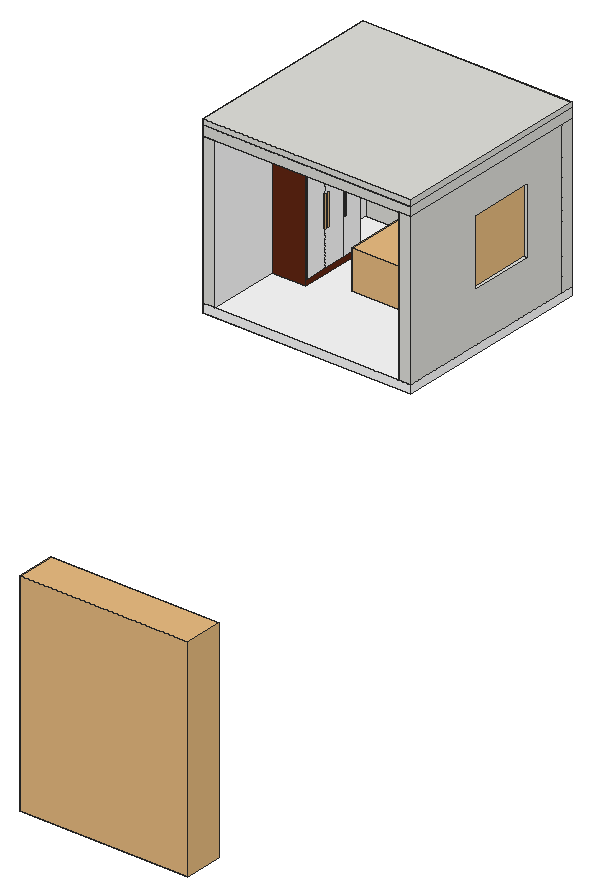
# SketchUp Ruby script. Lengths in inches.
U = 1.inch
M = Sketchup.active_model
def pt(a) = Geom::Point3d.new(a.map { |v| v * U })
def face(e, loops, mat)
  f = e.add_face(loops[0].map { |a| pt(a) })
  loops[1..].each { |l| e.add_face(l.map { |a| pt(a) }).erase! }
  f.material = f.back_material = mat if mat
  f
end
# faces: each face lists its corners as indices into pts; further lists are holes
def faces(e, pts, list, mat = nil) = list.each { |f| face(e, (f[0].is_a?(Array) ? f : [f]).map { |l| l.map { |i| pts[i] } }, mat) }
# xy, xz, yz: faces in a plane at the given z, y or x. An outline is a flat list of corners, or four numbers for a rectangle; further outlines are holes
def ring(l) = l.size == 4 ? [[l[0], l[1]], [l[2], l[1]], [l[2], l[3]], [l[0], l[3]]] : l.each_slice(2).to_a
def flat(e, list, mat, &to3) = list.each { |f| face(e, (f[0].is_a?(Array) ? f : [f]).map { |l| ring(l).map { |u, v| to3.(u, v) } }, mat) }
def xy(e, z, list, mat = nil) = flat(e, list, mat) { |x, y| [x, y, z] }
def xz(e, y, list, mat = nil) = flat(e, list, mat) { |x, z| [x, y, z] }
def yz(e, x, list, mat = nil) = flat(e, list, mat) { |y, z| [x, y, z] }
def lines(e, pts, list) = list.each { |a, b| e.add_line(pt(pts[a]), pt(pts[b])) }
# prism: a flat outline (further loops are holes) pulled along v
def prism(e, loops, v, mat = nil)
  f = face(e, loops, mat); d = Geom::Vector3d.new(v.map { |x| x * U })
  f.pushpull(f.normal.samedirection?(d) ? d.length : -d.length)
end
def box(e, o, s, mat = nil) = prism(e, [[o, [o[0] + s[0], o[1], o[2]], [o[0] + s[0], o[1] + s[1], o[2]], [o[0], o[1] + s[1], o[2]]]], [0, 0, s[2]], mat)
def at(x, y, z, deg = 0) = Geom::Transformation.translation(pt([x, y, z])) * Geom::Transformation.rotation(ORIGIN, Z_AXIS, deg.degrees)
def axes(o, x, y, z) = Geom::Transformation.new([*x, 0, *y, 0, *z, 0, *pt(o).to_a, 1])
def part(name) = M.definitions.add(name)
# library, detail: a bought-in or finely detailed component or shape, given as its bounding box
def library(name, o, s) = part(name).tap { |d| box(d.entities, o, s) }
def detail(e, o, s) = box(e.add_group.entities, o, s)
def put(e, d, t, mat = nil) = e.add_instance(d, t).tap { |i| i.material = mat if mat }
def group(e, t, mat = nil) = e.add_group.tap { |g| g.transformation = t; g.material = mat if mat }.entities
root = M.entities
M.materials.add("Ceramic Sand 8.13cm").color = [255, 255, 255]
M.materials.add("Emissive").color = [255, 202, 141]
M.materials.add("Emissive\#1").color = [255, 201, 138]
M.materials.add("Marble White 501 36.79cm").color = [255, 255, 255]
M.materials.add("Marble White 601 37.77cm\#1").color = [255, 255, 255]
M.materials.add("Wood Dark 02 100cm\#1").color = [99, 39, 19]
M.materials.add("[Color M09]4").color = [0, 0, 0]
M.materials.add("tecido").color = [198, 192, 183]
c1 = part("232mm Slimline Handle")
detail(c1.entities,[0,0,0],[9.13,0.47,1.38])
c2 = library("Double bed set",[6.09,0.88,0],[81.44,100.66,42.94])
c3 = library("Roman blind",[0,0,0],[2.24,37.33,21.19])
c4 = library("Window Crafter Sliding 2",[0,-0.07,0],[48,3.52,48])
c5 = library("Tlon Light 650 Ceiling 152 007",[-12.8,-12.8,-3.78],[25.6,25.6,3.58])
c6 = library("alpha",[-9.58,-11.73,2.09],[20.31,19.05,9.62])
c7 = library("Group\#10",[0,0,9.46],[84,1,110.54])
c8 = library("Group\#9",[0,0,0],[15.0625,1.3125,59.625])
c9 = part("Group\#353")
detail(c9.entities,[0,0,0],[1.58,1.18,1.58])
detail(root,[303.51,0,24.09],[120.56,27.875,151.41])
put(root,c1,axes([34,609.46,59.9],[0,0,-2.46],[0,1,0],[1,0,0]),"[Color M09]4")
put(root,c1,axes([34,627.9375,59.84],[0,0,-2.46],[0,1,0],[1,0,0]),"[Color M09]4")
put(root,c1,axes([34,612.23,59.66],[0,0,-2.46],[0,1,0],[1,0,0]),"[Color M09]4")
put(root,c2,axes([56.36,683.34,6],[0,-0.87706,0],[0.72394,0,0],[0,0,0.65]))
put(root,c3,axes([138.76,600.57,61.6],[1,0,0],[0,1.29,0],[0,0,1.34]),"tecido")
put(root,c4,at(143.81,648.57,42,-90))
put(root,c5,axes([40.37,556.16,114],[0.2,0,0],[0,0.2,0],[0,0,0.2]))
put(root,c5,axes([135.87,556.16,114],[0.2,0,0],[0,0.2,0],[0,0,0.2]))
put(root,c5,axes([135.87,665.54,114],[0.2,0,0],[0,0.2,0],[0,0,0.2]))
put(root,c5,axes([40.37,665.54,114],[0.2,0,0],[0,0.2,0],[0,0,0.2]))
put(root,c6,axes([87.5,610.64,98.94],[1,0,0],[0,1,0],[0,0,1.467]))
g1 = group(root,at(0,543.57,0))
box(g1,[0,0,0],[150,144,6],"Marble White 601 37.77cm\#1")
g2 = group(root,at(0,543.57,6))
xy(g2,0,[[0,0,9,135]])
xy(g2,108,[[0,0,9,135]])
xz(g2,0,[[0,0,9,108]])
xz(g2,135,[[0,0,9,108]])
yz(g2,0,[[0,0,135,108]])
yz(g2,9,[[0,0,135,108]],"Ceramic Sand 8.13cm")
g3 = group(root,at(9,594.57,6))
g4 = group(g3,at(24,0,5.09))
xy(g4,0,[[0,0,1,16.32],[0,16.64,1,32.09],[0,32.41,1,48.02]])
xy(g4,77.08,[[0,83.29,1,84]])
xy(g4,77.5,[[0,16.32,1,16.64],[0,32.09,1,32.41],[0,48.02,1,83.29]])
xy(g4,78.21,[[0,17.07,1,17.38],[0,33.58,1,33.9],[0,50.1,1,50.42],[0.0625,66.62,1,66.93]])
xy(g4,102.91,[[0,0,1,17.07],[0,17.38,1,33.58],[0,33.9,1,50.1],[0,50.42,1,50.42,1,66.62,0.0625,66.62,0.0625,66.93,1,66.93,1,84,0,84]],"Wood Dark 02 100cm\#1")
xz(g4,0,[[0,0,1,102.91]],"Wood Dark 02 100cm\#1")
xz(g4,16.32,[[0,0,1,77.5]])
xz(g4,16.64,[[0,0,1,77.5]])
xz(g4,17.07,[[0,78.21,1,102.21],[0,102.21,1,102.91]])
xz(g4,17.38,[[0,78.21,1,102.21],[0,102.21,1,102.91]])
xz(g4,32.09,[[0,0,1,77.5]])
xz(g4,32.41,[[0,0,1,77.5]])
xz(g4,33.58,[[0,78.21,1,102.21],[0,102.21,1,102.91]])
xz(g4,33.9,[[0,78.21,1,102.21],[0,102.21,1,102.91]])
xz(g4,48.02,[[0,0,1,77.5]])
xz(g4,50.1,[[0,78.21,1,102.21],[0,102.21,1,102.91]])
xz(g4,50.42,[[0,78.21,1,102.21],[0,102.21,1,102.91]])
xz(g4,66.62,[[0.0625,78.21,1,102.21],[0.0625,102.21,1,102.91]])
xz(g4,66.93,[[0.0625,78.21,1,102.21],[0.0625,102.21,1,102.91]])
xz(g4,83.29,[[0,77.08,1,77.5]])
xz(g4,84,[[0,77.08,1,102.91]])
yz(g4,0,[[0,0,0,102.91,17.07,102.91,17.07,78.21,17.38,78.21,17.38,102.91,33.58,102.91,33.58,78.21,33.9,78.21,33.9,102.91,50.1,102.91,50.1,78.21,50.42,78.21,50.42,102.91,84,102.91,84,77.08,83.29,77.08,83.29,77.5,48.02,77.5,48.02,0,32.41,0,32.41,77.5,32.09,77.5,32.09,0,16.64,0,16.64,77.5,16.32,77.5,16.32,0]])
yz(g4,0.0625,[[66.62,78.21,66.93,102.91]])
yz(g4,1,[[83.29,77.08,84,102.21],[83.29,102.21,84,102.91]])
yz(g4,1,[[0.71,0,16.32,77.5],[16.64,0,32.09,77.5],[32.41,0,48.02,77.5],[0.71,78.21,17.07,102.21],[17.38,78.21,33.58,102.21],
  [33.9,78.21,50.1,102.21],[50.42,78.21,66.62,102.21],[66.93,78.21,83.29,102.21]],"Marble White 501 36.79cm")
yz(g4,1,[[0,0,0.71,102.21],[0.71,77.5,83.29,78.21],[0,102.21,0.71,102.91],[0.71,102.21,17.07,102.91],[17.38,102.21,33.58,102.91],
  [33.9,102.21,50.1,102.91],[50.42,102.21,66.62,102.91],[66.93,102.21,83.29,102.91]],"Wood Dark 02 100cm\#1")
p = [[0,84,77.23],[1,83.29,77.08]]
lines(g4,p,[[0,1]])
g5 = group(g3,at(0,0,0))
xy(g5,0,[[0,0,24,48]],"Wood Dark 02 100cm\#1")
xy(g5,82.3125,[[0,48,24,84]],"Wood Dark 02 100cm\#1")
xy(g5,108,[[0,0,24,84]],"Wood Dark 02 100cm\#1")
xz(g5,0,[[0,0,24,108]],"Wood Dark 02 100cm\#1")
xz(g5,48,[[0,0,24,82.3125]],"Wood Dark 02 100cm\#1")
xz(g5,84,[[0,82.3125,24,108]],"Wood Dark 02 100cm\#1")
yz(g5,0,[[0,0,0,108,84,108,84,82.3125,48,82.3125,48,0]],"Wood Dark 02 100cm\#1")
yz(g5,24,[[0,0,47.69,108],[47.69,0,48,108],[48,82.3125,84,108]],"Wood Dark 02 100cm\#1")
put(root,c7,axes([57,676.57,8.4],[1,0,0],[0,1,0],[0,0,0.88]),"Wood Dark 02 100cm\#1")
put(root,c8,axes([37.8125,676.26,29.3],[1,0,0],[0,1,0],[0,0,0.88]))
put(root,c9,axes([35.18,610.64,96.31],[0,-1,0],[-1,0,0],[0,0,-1]))
put(root,c9,axes([35.18,614.33,96.31],[0,-1,0],[-1,0,0],[0,0,-1]))
put(root,c9,axes([35.18,631.05,96.31],[0,-1,0],[-1,0,0],[0,0,-1]))
put(root,c9,axes([35.18,664.09,96.31],[0,-1,0],[-1,0,0],[0,0,-1]))
put(root,c9,axes([35.18,660.16,96.31],[0,-1,0],[-1,0,0],[0,0,-1]))
g6 = group(root,at(0,678.57,6))
box(g6,[0,0,0],[150,9,108])
g7 = group(root,at(141,543.57,6))
xy(g7,0,[[0,0,9,135]])
xy(g7,36,[[0,57,9,105]])
xy(g7,84,[[0,57,9,105]])
xy(g7,108,[[0,0,9,135]])
xz(g7,0,[[0,0,9,108]])
xz(g7,57,[[0,36,9,84]])
xz(g7,105,[[0,36,9,84]])
xz(g7,135,[[0,0,9,108]])
yz(g7,0,[[[0,0,135,108],[57,36,105,84]]],"Ceramic Sand 8.13cm")
yz(g7,9,[[[0,0,135,108],[57,36,105,84]]])
g8 = group(root,at(0,543.57,114))
xy(g8,0,[[0,0,0,144,150,144,150,0,141,0,141,134,34,134,34,0],[[34,0,141,134],[46,12,129,122]]])
xy(g8,2.125,[[58,24,117,110]])
xy(g8,4,[[[40.37,6.37,134.63,127.63],[46,12,129,122]],[[58,24,117,110],[62.67,28.67,112.33,105.33]]],"Emissive\#1")
xy(g8,7,[[[0,0,150,144],[40.37,6.37,134.63,127.63]],[62.67,28.67,112.33,105.33]])
xz(g8,0,[[0,0,150,7]])
xz(g8,6.37,[[40.37,4,134.63,7]])
xz(g8,12,[[46,0,129,4]])
xz(g8,24,[[58,2.125,117,4]])
xz(g8,28.67,[[62.67,4,112.33,7]])
xz(g8,105.33,[[62.67,4,112.33,7]])
xz(g8,110,[[58,2.125,117,4]])
xz(g8,122,[[46,0,129,4]])
xz(g8,127.63,[[40.37,4,134.63,7]])
xz(g8,144,[[0,0,150,7]])
yz(g8,0,[[0,0,144,7]])
yz(g8,40.37,[[6.37,4,127.63,7]])
yz(g8,46,[[12,0,122,4]])
yz(g8,58,[[24,2.125,110,4]])
yz(g8,62.67,[[28.67,4,105.33,7]])
yz(g8,112.33,[[28.67,4,105.33,7]])
yz(g8,117,[[24,2.125,110,4]])
yz(g8,129,[[12,0,122,4]])
yz(g8,134.63,[[6.37,4,127.63,7]])
yz(g8,150,[[0,0,144,7]])
g9 = group(root,at(0,543.57,121))
box(g9,[0,0,0],[150,144,4])
g10 = group(root,at(34,677.57,8.4))
xy(g10,0,[[0,0,107,1]])
xy(g10,105.6,[[0,0,107,1]])
xz(g10,0,[[0,0,107,0,107,1.13,105.69,8.18,105.61,8.76,105.52,9.32,105.43,9.89,105.33,10.45,105.22,11.02,104.98,12.14,104.85,12.7,104.71,13.26,104.5625,13.8125,104.41,14.37,104.09,15.47,103.92,16.03,103.74,16.57,103.36,17.67,103.16,18.21,102.74,19.29,102.52,19.83,102.29,20.36,102.06,20.9,101.82,21.43,101.57,21.96,101.3125,22.48,101.05,23,100.79,23.53,100.51,24.04,100.23,24.56,99.95,25.07,99.35,26.09,99.05,26.59,98.74,27.09,98.42,27.59,98.09,28.09,97.43,29.07,96.38,30.51,96.02,30.98,95.65,31.46,95.28,31.92,94.9,32.39,94.51,32.85,94.12,33.3,93.73,33.76,93.32,34.2,92.92,34.65,92.08,35.53,91.66,35.96,91.23,36.39,90.8,36.8125,90.36,37.23,89.91,37.65,89.46,38.06,89,38.46,88.54,38.87,88.08,39.26,87.61,39.66,87.13,40.05,86.65,40.43,86.16,40.81,85.18,41.55,84.68,41.92,84.17,42.28,83.67,42.63,83.15,42.98,82.64,43.33,82.11,43.67,81.59,44,81.06,44.33,80.52,44.66,79.98,44.98,78.9,45.6,78.35,45.9,77.79,46.2,76.67,46.78,76.11,47.0625,75.54,47.34,74.97,47.61,73.23,48.39,72.65,48.63,72.06,48.875,71.47,49.11,70.28,49.57,69.68,49.79,69.08,50,68.47,50.21,67.86,50.41,66.03,50.98,65.41,51.15,64.79,51.33,63.55,51.65,62.29,51.95,61.03,52.23,60.4,52.36,59.77,52.48,58.49,52.7,57.86,52.81,57.22,52.91,56.58,53,55.93,53.08,55.29,53.16,54.64,53.24,54.2,53.29,53.75,53.34,53.3,53.4,52.85,53.47,52.41,53.54,51.96,53.61,51.52,53.69,51.08,53.78,50.63,53.86,49.75,54.06,49.32,54.16,48.88,54.27,48.45,54.38,48.01,54.5,47.15,54.74,46.72,54.87,46.3,55.01,45.87,55.15,45.45,55.29,44.61,55.59,44.19,55.75,43.78,55.91,42.55,56.42,42.15,56.6,41.74,56.79,41.34,56.97,40.95,57.17,40.55,57.36,40.16,57.5625,39.77,57.77,39.38,57.98,39,58.1875,38.62,58.41,38.24,58.625,37.87,58.85,37.5,59.08,37.13,59.3125,36.77,59.55,36.4,59.79,36.05,60.03,35.69,60.28,35.34,60.53,34.99,60.79,34.65,61.05,34.31,61.3125,33.97,61.58,33.31,62.12,32.98,62.4,32.34,62.96,31.41,63.83,30.81,64.43,30.51,64.74,30.22,65.04,29.9375,65.35,29.66,65.66,29.38,65.98,28.84,66.62,28.58,66.94,28.32,67.27,28.0625,67.6,27.81,67.93,27.5625,68.27,27.32,68.6,27.09,68.94,26.85,69.29,26.63,69.63,26.41,69.98,26.1875,70.33,25.97,70.68,25.77,71.04,25.5625,71.39,25.37,71.75,25.17,72.11,24.98,72.47,24.62,73.21,24.45,73.57,24.28,73.94,24.12,74.32,23.96,74.69,23.81,75.07,23.66,75.44,23.38,76.2,23.25,76.58,23.12,76.97,23,77.35,22.88,77.74,22.77,78.12,22.47,79.29,22.38,79.68,22.22,80.46,22.14,80.86,22.08,81.25,22.01,81.65,21.96,82.04,21.9,82.4375,21.86,82.83,21.78,83.63,21.75,84.03,21.73,84.43,21.71,84.82,21.69,85.22,21.69,85.62,21.68,86.02,21.68,105.6,0,105.6]],"Ceramic Sand 8.13cm")
xz(g10,0,[[107,1.13,107,8.33,106.92,8.91,106.83,9.49,106.73,10.0625,106.625,10.64,106.51,11.22,106.4,11.79,106.27,12.36,106.14,12.9375,105.99,13.51,105.85,14.08,105.69,14.65,105.53,15.21,105.36,15.78,105,16.9,104.8125,17.46,104.61,18.02,104.41,18.57,104.2,19.13,103.98,19.68,103.52,20.78,103.04,21.86,102.26,23.48,101.7,24.54,101.42,25.06,101.125,25.59,100.83,26.11,100.52,26.63,100.21,27.14,99.89,27.66,99.5625,28.17,99.23,28.67,98.55,29.67,98.2,30.17,97.48,31.15,97.11,31.64,96.73,32.12,96.35,32.59,95.96,33.07,95.57,33.54,95.17,34.01,94.35,34.93,93.9375,35.38,93.51,35.83,93.09,36.28,92.21,37.16,91.77,37.59,91.32,38.02,90.86,38.45,90.4,38.87,89.9375,39.28,89.47,39.69,88.99,40.1,88.51,40.5,88.02,40.9,87.53,41.29,87.03,41.68,86.53,42.0625,86.03,42.44,85.51,42.81,85,43.18,84.48,43.55,83.95,43.9,83.43,44.26,82.89,44.6,82.35,44.95,81.8125,45.28,81.27,45.61,80.71,45.94,80.16,46.26,79.6,46.58,79.04,46.89,77.33,47.79,76.75,48.07,76.17,48.36,75.59,48.63,74.41,49.17,73.8125,49.43,73.21,49.68,72.61,49.93,72.01,50.17,71.4,50.41,70.79,50.64,70.18,50.86,69.5625,51.08,68.94,51.29,68.32,51.5,67.7,51.7,66.44,52.08,65.8125,52.26,65.18,52.43,64.54,52.6,63.91,52.77,63.27,52.92,61.98,53.22,61.34,53.35,60.69,53.49,59.39,53.73,58.09,53.95,57.43,54.05,56.78,54.14,56.125,54.23,55.47,54.3125,54.81,54.39,54.375,54.43,53.94,54.49,53.08,54.61,52.22,54.75,51.36,54.91,50.94,54.99,50.51,55.08,50.09,55.18,49.66,55.28,49.24,55.38,48.82,55.49,48.41,55.6,47.57,55.84,46.34,56.23,45.93,56.37,45.53,56.51,45.12,56.66,44.72,56.8125,44.32,56.97,43.92,57.13,43.53,57.29,43.14,57.46,42.74,57.64,42.36,57.8125,41.97,57.99,41.21,58.37,40.83,58.5625,40.45,58.76,40.08,58.96,39.71,59.17,39.34,59.375,38.98,59.59,38.26,60.03,37.91,60.25,37.55,60.48,37.21,60.71,36.86,60.95,36.52,61.1875,36.18,61.43,35.84,61.68,35.18,62.18,34.86,62.4375,34.53,62.7,34.22,62.96,33.9,63.23,33.28,63.77,32.68,64.33,32.39,64.61,32.09,64.9,31.81,65.19,31.52,65.48,31.24,65.78,30.43,66.68,30.16,66.99,29.91,67.3,29.65,67.61,29.15,68.25,28.91,68.57,28.68,68.89,28.44,69.22,28.21,69.54,27.77,70.21,27.56,70.54,27.14,71.22,26.94,71.5625,26.74,71.91,26.55,72.25,26.01,73.3,25.84,73.66,25.67,74.01,25.35,74.73,25.05,75.45,24.91,75.8125,24.77,76.18,24.64,76.55,24.51,76.91,24.27,77.65,24.16,78.03,24.05,78.4,23.95,78.77,23.85,79.15,23.76,79.52,23.67,79.9,23.59,80.28,23.38,81.42,23.26,82.18,23.21,82.5625,23.17,82.95,23.09,83.71,23.07,84.1,23.04,84.48,23.02,84.87,23.01,85.25,23,85.64,23,105.6,21.68,105.6,21.68,86.02,21.69,85.62,21.69,85.22,21.71,84.82,21.73,84.43,21.75,84.03,21.78,83.63,21.86,82.83,21.9,82.4375,21.96,82.04,22.01,81.65,22.08,81.25,22.14,80.86,22.22,80.46,22.38,79.68,22.47,79.29,22.77,78.12,22.88,77.74,23,77.35,23.12,76.97,23.25,76.58,23.38,76.2,23.66,75.44,23.81,75.07,23.96,74.69,24.12,74.32,24.28,73.94,24.45,73.57,24.62,73.21,24.98,72.47,25.17,72.11,25.37,71.75,25.5625,71.39,25.77,71.04,25.97,70.68,26.1875,70.33,26.41,69.98,26.63,69.63,26.85,69.29,27.09,68.94,27.32,68.6,27.5625,68.27,27.81,67.93,28.0625,67.6,28.32,67.27,28.58,66.94,28.84,66.62,29.38,65.98,29.66,65.66,29.9375,65.35,30.22,65.04,30.51,64.74,30.81,64.43,31.41,63.83,32.34,62.96,32.98,62.4,33.31,62.12,33.97,61.58,34.31,61.3125,34.65,61.05,34.99,60.79,35.34,60.53,35.69,60.28,36.05,60.03,36.4,59.79,36.77,59.55,37.13,59.3125,37.5,59.08,37.87,58.85,38.24,58.625,38.62,58.41,39,58.1875,39.38,57.98,39.77,57.77,40.16,57.5625,40.55,57.36,40.95,57.17,41.34,56.97,41.74,56.79,42.15,56.6,42.55,56.42,43.78,55.91,44.19,55.75,44.61,55.59,45.45,55.29,45.87,55.15,46.3,55.01,46.72,54.87,47.15,54.74,48.01,54.5,48.45,54.38,48.88,54.27,49.32,54.16,49.75,54.06,50.63,53.86,51.08,53.78,51.52,53.69,51.96,53.61,52.41,53.54,52.85,53.47,53.3,53.4,53.75,53.34,54.2,53.29,54.64,53.24,55.29,53.16,55.93,53.08,56.58,53,57.22,52.91,57.86,52.81,58.49,52.7,59.77,52.48,60.4,52.36,61.03,52.23,62.29,51.95,63.55,51.65,64.79,51.33,65.41,51.15,66.03,50.98,67.86,50.41,68.47,50.21,69.08,50,69.68,49.79,70.28,49.57,71.47,49.11,72.06,48.875,72.65,48.63,73.23,48.39,74.97,47.61,75.54,47.34,76.11,47.0625,76.67,46.78,77.79,46.2,78.35,45.9,78.9,45.6,79.98,44.98,80.52,44.66,81.06,44.33,81.59,44,82.11,43.67,82.64,43.33,83.15,42.98,83.67,42.63,84.17,42.28,84.68,41.92,85.18,41.55,86.16,40.81,86.65,40.43,87.13,40.05,87.61,39.66,88.08,39.26,88.54,38.87,89,38.46,89.46,38.06,89.91,37.65,90.36,37.23,90.8,36.8125,91.23,36.39,91.66,35.96,92.08,35.53,92.92,34.65,93.32,34.2,93.73,33.76,94.12,33.3,94.51,32.85,94.9,32.39,95.28,31.92,95.65,31.46,96.02,30.98,96.38,30.51,97.43,29.07,98.09,28.09,98.42,27.59,98.74,27.09,99.05,26.59,99.35,26.09,99.95,25.07,100.23,24.56,100.51,24.04,100.79,23.53,101.05,23,101.3125,22.48,101.57,21.96,101.82,21.43,102.06,20.9,102.29,20.36,102.52,19.83,102.74,19.29,103.16,18.21,103.36,17.67,103.74,16.57,103.92,16.03,104.09,15.47,104.41,14.37,104.5625,13.8125,104.71,13.26,104.85,12.7,104.98,12.14,105.22,11.02,105.33,10.45,105.43,9.89,105.52,9.32,105.61,8.76,105.69,8.18]],"Emissive")
xz(g10,0,[[107,8.33,107,105.6,23,105.6,23,85.64,23.01,85.25,23.02,84.87,23.04,84.48,23.07,84.1,23.09,83.71,23.17,82.95,23.21,82.5625,23.26,82.18,23.38,81.42,23.59,80.28,23.67,79.9,23.76,79.52,23.85,79.15,23.95,78.77,24.05,78.4,24.16,78.03,24.27,77.65,24.51,76.91,24.64,76.55,24.77,76.18,24.91,75.8125,25.05,75.45,25.35,74.73,25.67,74.01,25.84,73.66,26.01,73.3,26.55,72.25,26.74,71.91,26.94,71.5625,27.14,71.22,27.56,70.54,27.77,70.21,28.21,69.54,28.44,69.22,28.68,68.89,28.91,68.57,29.15,68.25,29.65,67.61,29.91,67.3,30.16,66.99,30.43,66.68,31.24,65.78,31.52,65.48,31.81,65.19,32.09,64.9,32.39,64.61,32.68,64.33,33.28,63.77,33.9,63.23,34.22,62.96,34.53,62.7,34.86,62.4375,35.18,62.18,35.84,61.68,36.18,61.43,36.52,61.1875,36.86,60.95,37.21,60.71,37.55,60.48,37.91,60.25,38.26,60.03,38.98,59.59,39.34,59.375,39.71,59.17,40.08,58.96,40.45,58.76,40.83,58.5625,41.21,58.37,41.97,57.99,42.36,57.8125,42.74,57.64,43.14,57.46,43.53,57.29,43.92,57.13,44.32,56.97,44.72,56.8125,45.12,56.66,45.53,56.51,45.93,56.37,46.34,56.23,47.57,55.84,48.41,55.6,48.82,55.49,49.24,55.38,49.66,55.28,50.09,55.18,50.51,55.08,50.94,54.99,51.36,54.91,52.22,54.75,53.08,54.61,53.94,54.49,54.375,54.43,54.81,54.39,55.47,54.3125,56.125,54.23,56.78,54.14,57.43,54.05,58.09,53.95,59.39,53.73,60.69,53.49,61.34,53.35,61.98,53.22,63.27,52.92,63.91,52.77,64.54,52.6,65.18,52.43,65.8125,52.26,66.44,52.08,67.7,51.7,68.32,51.5,68.94,51.29,69.5625,51.08,70.18,50.86,70.79,50.64,71.4,50.41,72.01,50.17,72.61,49.93,73.21,49.68,73.8125,49.43,74.41,49.17,75.59,48.63,76.17,48.36,76.75,48.07,77.33,47.79,79.04,46.89,79.6,46.58,80.16,46.26,80.71,45.94,81.27,45.61,81.8125,45.28,82.35,44.95,82.89,44.6,83.43,44.26,83.95,43.9,84.48,43.55,85,43.18,85.51,42.81,86.03,42.44,86.53,42.0625,87.03,41.68,87.53,41.29,88.02,40.9,88.51,40.5,88.99,40.1,89.47,39.69,89.9375,39.28,90.4,38.87,90.86,38.45,91.32,38.02,91.77,37.59,92.21,37.16,93.09,36.28,93.51,35.83,93.9375,35.38,94.35,34.93,95.17,34.01,95.57,33.54,95.96,33.07,96.35,32.59,96.73,32.12,97.11,31.64,97.48,31.15,98.2,30.17,98.55,29.67,99.23,28.67,99.5625,28.17,99.89,27.66,100.21,27.14,100.52,26.63,100.83,26.11,101.125,25.59,101.42,25.06,101.7,24.54,102.26,23.48,103.04,21.86,103.52,20.78,103.98,19.68,104.2,19.13,104.41,18.57,104.61,18.02,104.8125,17.46,105,16.9,105.36,15.78,105.53,15.21,105.69,14.65,105.85,14.08,105.99,13.51,106.14,12.9375,106.27,12.36,106.4,11.79,106.51,11.22,106.625,10.64,106.73,10.0625,106.83,9.49,106.92,8.91]],"Wood Dark 02 100cm\#1")
xz(g10,1,[[0,0,107,105.6]])
yz(g10,0,[[0,0,1,105.6]])
yz(g10,107,[[0,0,1,105.6]])
p = [[108.33,0,9.67],[108.42,0,9.08],[108.5,0,8.49],[107,0,15.53],[107.16,0,14.96],[107.32,0,14.38],
  [108.12,0,10.86],[108.23,0,10.27],[107.88,0,12.04],[108.01,0,11.45],[107.75,0,12.625],[107.62,0,13.21],
  [107.47,0,13.8]]
lines(g10,p,[[0,1],[1,2],[3,4],[4,5],[6,7],[8,9],[7,0],[10,8],[11,10],[9,6],[5,12],[12,11]])
